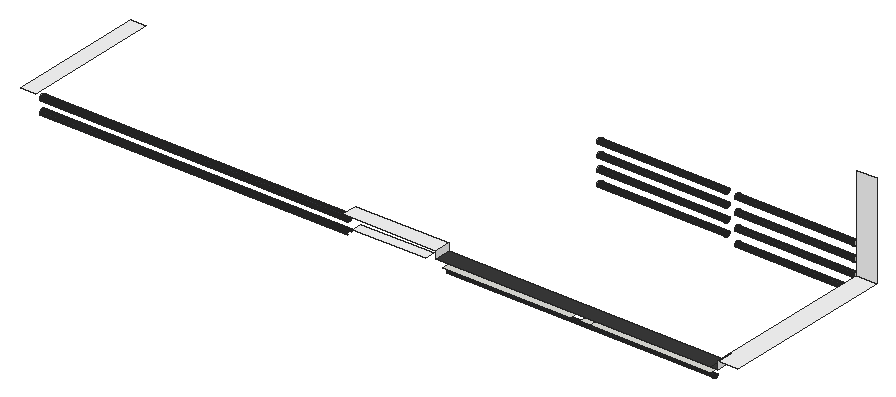
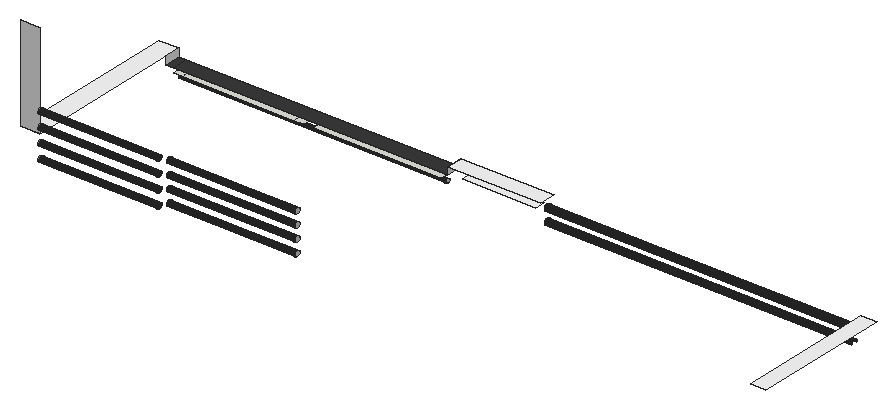
# SketchUp Ruby script. Lengths in inches.
U = 1.inch
M = Sketchup.active_model
def pt(a) = Geom::Point3d.new(a.map { |v| v * U })
def face(e, loops, mat)
  f = e.add_face(loops[0].map { |a| pt(a) })
  loops[1..].each { |l| e.add_face(l.map { |a| pt(a) }).erase! }
  f.material = f.back_material = mat if mat
  f
end
# faces: each face lists its corners as indices into pts; further lists are holes
def faces(e, pts, list, mat = nil) = list.each { |f| face(e, (f[0].is_a?(Array) ? f : [f]).map { |l| l.map { |i| pts[i] } }, mat) }
# xy, xz, yz: faces in a plane at the given z, y or x. An outline is a flat list of corners, or four numbers for a rectangle; further outlines are holes
def ring(l) = l.size == 4 ? [[l[0], l[1]], [l[2], l[1]], [l[2], l[3]], [l[0], l[3]]] : l.each_slice(2).to_a
def flat(e, list, mat, &to3) = list.each { |f| face(e, (f[0].is_a?(Array) ? f : [f]).map { |l| ring(l).map { |u, v| to3.(u, v) } }, mat) }
def xy(e, z, list, mat = nil) = flat(e, list, mat) { |x, y| [x, y, z] }
def xz(e, y, list, mat = nil) = flat(e, list, mat) { |x, z| [x, y, z] }
def yz(e, x, list, mat = nil) = flat(e, list, mat) { |y, z| [x, y, z] }
def lines(e, pts, list) = list.each { |a, b| e.add_line(pt(pts[a]), pt(pts[b])) }
# prism: a flat outline (further loops are holes) pulled along v
def prism(e, loops, v, mat = nil)
  f = face(e, loops, mat); d = Geom::Vector3d.new(v.map { |x| x * U })
  f.pushpull(f.normal.samedirection?(d) ? d.length : -d.length)
end
def box(e, o, s, mat = nil) = prism(e, [[o, [o[0] + s[0], o[1], o[2]], [o[0] + s[0], o[1] + s[1], o[2]], [o[0], o[1] + s[1], o[2]]]], [0, 0, s[2]], mat)
def at(x, y, z, deg = 0) = Geom::Transformation.translation(pt([x, y, z])) * Geom::Transformation.rotation(ORIGIN, Z_AXIS, deg.degrees)
def axes(o, x, y, z) = Geom::Transformation.new([*x, 0, *y, 0, *z, 0, *pt(o).to_a, 1])
def part(name) = M.definitions.add(name)
# library, detail: a bought-in or finely detailed component or shape, given as its bounding box
def library(name, o, s) = part(name).tap { |d| box(d.entities, o, s) }
def detail(e, o, s) = box(e.add_group.entities, o, s)
def put(e, d, t, mat = nil) = e.add_instance(d, t).tap { |i| i.material = mat if mat }
def group(e, t, mat = nil) = e.add_group.tap { |g| g.transformation = t; g.material = mat if mat }.entities
root = M.entities
M.materials.add("[Carrera Marble]").color = [252, 252, 252]
M.materials.add("[Color M07]").color = [58, 58, 58]
M.materials.add("[Formica Laminate Dark]").color = [50, 53, 60]
xy(root,65.34,[[464.36,270.82,564.04,283.23],[571.61,270.82,579.17,283.23],[579.17,270.82,673.42,283.23]])
xy(root,67.32,[[394.4,270.82,451.35,278.69]],"[Carrera Marble]")
xy(root,69.375,[[459.28,270.82,673.42,283.23],[673.42,270.82,679.23,283.23]],"[Color M07]")
xy(root,75.25,[[134.55,270.82,146.33,378.85],[386.47,270.82,459.28,283.23],[679.23,270.82,694.52,406.29]],"[Carrera Marble]")
xz(root,406.29,[[679.23,75.25,694.52,149.125]],"[Carrera Marble]")
yz(root,146.33,[[277.43,67.33,276.8,67.41,276.21,67.65,275.71,68.04,275.32,68.54,275.08,69.13,274.99,69.76,275.08,70.39,275.32,70.98,275.71,71.49,276.21,71.875,276.8,72.12,277.43,72.2,278.0625,72.12,278.65,71.875,279.15,71.49,279.54,70.98,279.78,70.39,279.87,69.76,279.78,69.13,279.54,68.54,279.15,68.04,278.65,67.65,278.0625,67.41]])
yz(root,459.28,[[270.82,69.375,283.23,75.25]],"[Carrera Marble]")
yz(root,464.36,[[276.43,59.2,276.06,59.25,275.71,59.4,275.41,59.625,275.18,59.92,275.04,60.27,274.99,60.64,275.04,61.01,275.18,61.36,275.41,61.66,275.71,61.89,276.06,62.03,276.43,62.08,276.8,62.03,277.15,61.89,277.44,61.66,277.67,61.36,277.82,61.01,277.87,60.64,277.82,60.27,277.67,59.92,277.44,59.625,277.15,59.4,276.8,59.25]])
yz(root,473.77,[[411.5,63.75,411,63.8125,410.53,64.01,410.13,64.32,409.82,64.72,409.63,65.18,409.5625,65.6875,409.63,66.1875,409.82,66.65,410.13,67.06,410.53,67.36,411,67.56,411.5,67.625,412,67.56,412.47,67.36,412.87,67.06,413.18,66.65,413.37,66.1875,413.4375,65.6875,413.37,65.18,413.18,64.72,412.87,64.32,412.47,64.01,412,63.8125],[411.5,73.75,411,73.8125,410.53,74.01,410.13,74.32,409.82,74.72,409.63,75.18,409.5625,75.6875,409.63,76.1875,409.82,76.65,410.13,77.06,410.53,77.36,411,77.56,411.5,77.625,412,77.56,412.47,77.36,412.87,77.06,413.18,76.65,413.37,76.1875,413.4375,75.6875,413.37,75.18,413.18,74.72,412.87,74.32,412.47,74.01,412,73.8125],[411.5,83.75,411,83.8125,410.53,84.01,410.13,84.32,409.82,84.72,409.63,85.18,409.5625,85.6875,409.63,86.1875,409.82,86.65,410.13,87.06,410.53,87.36,411,87.56,411.5,87.625,412,87.56,412.47,87.36,412.87,87.06,413.18,86.65,413.37,86.1875,413.4375,85.6875,413.37,85.18,413.18,84.72,412.87,84.32,412.47,84.01,412,83.8125],[411.5,93.75,411,93.8125,410.53,94.01,410.13,94.32,409.82,94.72,409.63,95.18,409.5625,95.6875,409.63,96.1875,409.82,96.65,410.13,97.06,410.53,97.36,411,97.56,411.5,97.625,412,97.56,412.47,97.36,412.87,97.06,413.18,96.65,413.37,96.1875,413.4375,95.6875,413.37,95.18,413.18,94.72,412.87,94.32,412.47,94.01,412,93.8125]])
yz(root,674.94,[[411.43,59.33,411.93,59.4,412.39,59.59,412.8,59.9,413.1,60.3,413.3,60.77,413.36,61.27,413.3,61.77,413.1,62.24,412.8,62.64,412.39,62.95,411.93,63.14,411.43,63.21,410.92,63.14,410.46,62.95,410.06,62.64,409.75,62.24,409.55,61.77,409.49,61.27,409.55,60.77,409.75,60.3,410.06,59.9,410.46,59.59,410.92,59.4],[411.43,70.46,411.93,70.52,412.39,70.72,412.8,71.02,413.1,71.43,413.3,71.89,413.36,72.39,413.3,72.9,413.1,73.36,412.8,73.76,412.39,74.07,411.93,74.27,411.43,74.33,410.92,74.27,410.46,74.07,410.06,73.76,409.75,73.36,409.55,72.9,409.49,72.39,409.55,71.89,409.75,71.43,410.06,71.02,410.46,70.72,410.92,70.52],[411.43,81.58,411.93,81.65,412.39,81.84,412.8,82.15,413.1,82.55,413.3,83.02,413.36,83.52,413.3,84.02,413.1,84.49,412.8,84.89,412.39,85.2,411.93,85.39,411.43,85.46,410.92,85.39,410.46,85.2,410.06,84.89,409.75,84.49,409.55,84.02,409.49,83.52,409.55,83.02,409.75,82.55,410.06,82.15,410.46,81.84,410.92,81.65],[411.43,92.71,411.93,92.77,412.39,92.97,412.8,93.27,413.1,93.68,413.3,94.14,413.36,94.64,413.3,95.15,413.1,95.61,412.8,96.01,412.39,96.32,411.93,96.52,411.43,96.58,410.92,96.52,410.46,96.32,410.06,96.01,409.75,95.61,409.55,95.15,409.49,94.64,409.55,94.14,409.75,93.68,410.06,93.27,410.46,92.97,410.92,92.77]])
yz(root,679.23,[[270.82,69.375,283.23,75.25]],"[Carrera Marble]")
p = [[146.33,274.99,59.45],[146.33,275.08,58.82],[386.47,275.08,58.82],[386.47,274.99,59.45],[146.33,279.78,58.82],[146.33,279.87,59.45],
  [386.47,279.87,59.45],[386.47,279.78,58.82],[464.36,276.06,59.25],[464.36,276.43,59.2],[673.42,276.43,59.2],[673.42,276.06,59.25],
  [464.36,276.8,59.25],[673.42,276.8,59.25],[464.36,275.71,59.4],[673.42,275.71,59.4],[464.36,277.15,59.4],[673.42,277.15,59.4],
  [674.94,411.43,59.33],[674.94,410.92,59.4],[581.54,410.92,59.4],[581.54,411.43,59.33],[674.94,411.93,59.4],[581.54,411.93,59.4],
  [464.36,275.41,59.625],[673.42,275.41,59.625],[464.36,277.44,59.625],[673.42,277.44,59.625],[674.94,410.46,59.59],[581.54,410.46,59.59],
  [674.94,412.39,59.59],[581.54,412.39,59.59],[146.33,275.08,60.08],[386.47,275.08,60.08],[146.33,279.78,60.08],[386.47,279.78,60.08],
  [464.36,275.18,59.92],[673.42,275.18,59.92],[464.36,277.67,59.92],[673.42,277.67,59.92],[674.94,410.06,59.9],[581.54,410.06,59.9],
  [674.94,412.8,59.9],[581.54,412.8,59.9],[464.36,275.04,60.27],[673.42,275.04,60.27],[464.36,277.82,60.27],[673.42,277.82,60.27],
  [674.94,409.75,60.3],[581.54,409.75,60.3],[674.94,413.1,60.3],[581.54,413.1,60.3],[146.33,275.32,60.67],[386.47,275.32,60.67],
  [146.33,279.54,60.67],[386.47,279.54,60.67],[464.36,274.99,60.64],[673.42,274.99,60.64],[464.36,277.87,60.64],[673.42,277.87,60.64],
  [674.94,409.55,60.77],[581.54,409.55,60.77],[674.94,413.3,60.77],[581.54,413.3,60.77],[464.36,275.04,61.01],[673.42,275.04,61.01],
  [464.36,277.82,61.01],[673.42,277.82,61.01],[146.33,275.71,61.17],[386.47,275.71,61.17],[146.33,279.15,61.17],[386.47,279.15,61.17],
  [674.94,409.49,61.27],[581.54,409.49,61.27],[674.94,413.36,61.27],[581.54,413.36,61.27],[464.36,275.18,61.36],[673.42,275.18,61.36],
  [464.36,277.67,61.36],[673.42,277.67,61.36],[146.33,276.21,61.5625],[386.47,276.21,61.5625],[146.33,278.65,61.5625],[386.47,278.65,61.5625],
  [674.94,409.55,61.77],[581.54,409.55,61.77],[674.94,413.3,61.77],[581.54,413.3,61.77],[464.36,275.41,61.66],[673.42,275.41,61.66],
  [464.36,277.44,61.66],[673.42,277.44,61.66],[146.33,276.8,61.8],[386.47,276.8,61.8],[146.33,278.0625,61.8],[386.47,278.0625,61.8],
  [464.36,275.71,61.89],[673.42,275.71,61.89],[464.36,277.15,61.89],[673.42,277.15,61.89],[146.33,277.43,61.89],[386.47,277.43,61.89],
  [674.94,409.75,62.24],[581.54,409.75,62.24],[674.94,413.1,62.24],[581.54,413.1,62.24],[464.36,276.06,62.03],[673.42,276.06,62.03],
  [464.36,276.8,62.03],[673.42,276.8,62.03],[464.36,276.43,62.08],[673.42,276.43,62.08],[674.94,410.06,62.64],[581.54,410.06,62.64],
  [674.94,412.8,62.64],[581.54,412.8,62.64],[674.94,410.46,62.95],[581.54,410.46,62.95],[674.94,412.39,62.95],[581.54,412.39,62.95],
  [674.94,410.92,63.14],[581.54,410.92,63.14],[674.94,411.93,63.14],[581.54,411.93,63.14],[674.94,411.43,63.21],[581.54,411.43,63.21],
  [473.77,411,63.8125],[473.77,411.5,63.75],[574.36,411.5,63.75],[574.36,411,63.8125],[473.77,412,63.8125],[574.36,412,63.8125],
  [473.77,410.53,64.01],[574.36,410.53,64.01],[473.77,412.47,64.01],[574.36,412.47,64.01],[473.77,410.13,64.32],[574.36,410.13,64.32],
  [473.77,412.87,64.32],[574.36,412.87,64.32],[473.77,409.82,64.72],[574.36,409.82,64.72],[473.77,413.18,64.72],[574.36,413.18,64.72],
  [473.77,409.63,65.18],[574.36,409.63,65.18],[473.77,413.37,65.18],[574.36,413.37,65.18],[473.77,409.5625,65.6875],[574.36,409.5625,65.6875],
  [473.77,413.4375,65.6875],[574.36,413.4375,65.6875],[473.77,409.63,66.1875],[574.36,409.63,66.1875],[473.77,413.37,66.1875],[574.36,413.37,66.1875],
  [473.77,409.82,66.65],[574.36,409.82,66.65],[473.77,413.18,66.65],[574.36,413.18,66.65],[473.77,410.13,67.06],[574.36,410.13,67.06],
  [473.77,412.87,67.06],[574.36,412.87,67.06],[473.77,410.53,67.36],[574.36,410.53,67.36],[473.77,412.47,67.36],[574.36,412.47,67.36],
  [146.33,276.8,67.41],[146.33,277.43,67.33],[386.47,277.43,67.33],[386.47,276.8,67.41],[146.33,278.0625,67.41],[386.47,278.0625,67.41],
  [146.33,276.21,67.65],[386.47,276.21,67.65],[146.33,278.65,67.65],[386.47,278.65,67.65],[473.77,411,67.56],[574.36,411,67.56],
  [473.77,412,67.56],[574.36,412,67.56],[473.77,411.5,67.625],[574.36,411.5,67.625],[146.33,275.71,68.04],[386.47,275.71,68.04],
  [146.33,279.15,68.04],[386.47,279.15,68.04],[146.33,275.32,68.54],[386.47,275.32,68.54],[146.33,279.54,68.54],[386.47,279.54,68.54],
  [146.33,275.08,69.13],[386.47,275.08,69.13],[146.33,279.78,69.13],[386.47,279.78,69.13],[146.33,274.99,69.76],[386.47,274.99,69.76],
  [146.33,279.87,69.76],[386.47,279.87,69.76],[146.33,275.08,70.39],[386.47,275.08,70.39],[146.33,279.78,70.39],[386.47,279.78,70.39],
  [146.33,275.32,70.98],[386.47,275.32,70.98],[146.33,279.54,70.98],[386.47,279.54,70.98],[674.94,410.92,70.52],[674.94,410.46,70.72],
  [581.54,410.46,70.72],[581.54,410.92,70.52],[674.94,411.43,70.46],[581.54,411.43,70.46],[674.94,411.93,70.52],[581.54,411.93,70.52],
  [674.94,412.39,70.72],[581.54,412.39,70.72],[674.94,410.06,71.02],[581.54,410.06,71.02],[674.94,412.8,71.02],[581.54,412.8,71.02],
  [146.33,275.71,71.49],[386.47,275.71,71.49],[146.33,279.15,71.49],[386.47,279.15,71.49],[674.94,409.75,71.43],[581.54,409.75,71.43],
  [674.94,413.1,71.43],[581.54,413.1,71.43],[674.94,409.55,71.89],[581.54,409.55,71.89],[674.94,413.3,71.89],[581.54,413.3,71.89],
  [146.33,276.21,71.875],[386.47,276.21,71.875],[146.33,278.65,71.875],[386.47,278.65,71.875],[146.33,276.8,72.12],[386.47,276.8,72.12],
  [146.33,278.0625,72.12],[386.47,278.0625,72.12],[674.94,409.49,72.39],[581.54,409.49,72.39],[674.94,413.36,72.39],[581.54,413.36,72.39],
  [146.33,277.43,72.2],[386.47,277.43,72.2],[674.94,409.55,72.9],[581.54,409.55,72.9],[674.94,413.3,72.9],[581.54,413.3,72.9],
  [674.94,409.75,73.36],[581.54,409.75,73.36],[674.94,413.1,73.36],[581.54,413.1,73.36],[674.94,410.06,73.76],[581.54,410.06,73.76],
  [674.94,412.8,73.76],[581.54,412.8,73.76],[473.77,411,73.8125],[473.77,411.5,73.75],[574.36,411.5,73.75],[574.36,411,73.8125],
  [473.77,412,73.8125],[574.36,412,73.8125],[674.94,410.46,74.07],[581.54,410.46,74.07],[473.77,410.53,74.01],[574.36,410.53,74.01],
  [473.77,412.47,74.01],[574.36,412.47,74.01],[674.94,412.39,74.07],[581.54,412.39,74.07],[473.77,410.13,74.32],[574.36,410.13,74.32],
  [473.77,412.87,74.32],[574.36,412.87,74.32],[674.94,410.92,74.27],[581.54,410.92,74.27],[674.94,411.93,74.27],[581.54,411.93,74.27],
  [473.77,409.82,74.72],[574.36,409.82,74.72],[674.94,411.43,74.33],[581.54,411.43,74.33],[473.77,413.18,74.72],[574.36,413.18,74.72],
  [473.77,409.63,75.18],[574.36,409.63,75.18],[473.77,413.37,75.18],[574.36,413.37,75.18],[473.77,409.5625,75.6875],[574.36,409.5625,75.6875],
  [473.77,413.4375,75.6875],[574.36,413.4375,75.6875],[473.77,409.63,76.1875],[574.36,409.63,76.1875],[473.77,413.37,76.1875],[574.36,413.37,76.1875],
  [473.77,409.82,76.65],[574.36,409.82,76.65],[473.77,413.18,76.65],[574.36,413.18,76.65],[473.77,410.13,77.06],[574.36,410.13,77.06],
  [473.77,412.87,77.06],[574.36,412.87,77.06],[473.77,410.53,77.36],[574.36,410.53,77.36],[473.77,412.47,77.36],[574.36,412.47,77.36],
  [473.77,411,77.56],[574.36,411,77.56],[473.77,412,77.56],[574.36,412,77.56],[473.77,411.5,77.625],[574.36,411.5,77.625],
  [674.94,410.92,81.65],[674.94,410.46,81.84],[581.54,410.46,81.84],[581.54,410.92,81.65],[674.94,411.43,81.58],[581.54,411.43,81.58],
  [674.94,411.93,81.65],[581.54,411.93,81.65],[674.94,412.39,81.84],[581.54,412.39,81.84],[674.94,410.06,82.15],[581.54,410.06,82.15],
  [674.94,412.8,82.15],[581.54,412.8,82.15],[674.94,409.75,82.55],[581.54,409.75,82.55],[674.94,413.1,82.55],[581.54,413.1,82.55],
  [674.94,409.55,83.02],[581.54,409.55,83.02],[674.94,413.3,83.02],[581.54,413.3,83.02],[674.94,409.49,83.52],[581.54,409.49,83.52],
  [674.94,413.36,83.52],[581.54,413.36,83.52],[674.94,409.55,84.02],[581.54,409.55,84.02],[674.94,413.3,84.02],[581.54,413.3,84.02],
  [473.77,411,83.8125],[473.77,411.5,83.75],[574.36,411.5,83.75],[574.36,411,83.8125],[473.77,412,83.8125],[574.36,412,83.8125],
  [473.77,410.53,84.01],[574.36,410.53,84.01],[473.77,412.47,84.01],[574.36,412.47,84.01],[674.94,409.75,84.49],[581.54,409.75,84.49],
  [473.77,410.13,84.32],[574.36,410.13,84.32],[473.77,412.87,84.32],[574.36,412.87,84.32],[674.94,413.1,84.49],[581.54,413.1,84.49],
  [473.77,409.82,84.72],[574.36,409.82,84.72],[473.77,413.18,84.72],[574.36,413.18,84.72],[674.94,410.06,84.89],[581.54,410.06,84.89],
  [674.94,412.8,84.89],[581.54,412.8,84.89],[473.77,409.63,85.18],[574.36,409.63,85.18],[473.77,413.37,85.18],[574.36,413.37,85.18],
  [674.94,410.46,85.2],[581.54,410.46,85.2],[674.94,412.39,85.2],[581.54,412.39,85.2],[473.77,409.5625,85.6875],[574.36,409.5625,85.6875],
  [674.94,410.92,85.39],[581.54,410.92,85.39],[674.94,411.93,85.39],[581.54,411.93,85.39],[473.77,413.4375,85.6875],[574.36,413.4375,85.6875],
  [674.94,411.43,85.46],[581.54,411.43,85.46],[473.77,409.63,86.1875],[574.36,409.63,86.1875],[473.77,413.37,86.1875],[574.36,413.37,86.1875],
  [473.77,409.82,86.65],[574.36,409.82,86.65],[473.77,413.18,86.65],[574.36,413.18,86.65],[473.77,410.13,87.06],[574.36,410.13,87.06],
  [473.77,412.87,87.06],[574.36,412.87,87.06],[473.77,410.53,87.36],[574.36,410.53,87.36],[473.77,412.47,87.36],[574.36,412.47,87.36],
  [473.77,411,87.56],[574.36,411,87.56],[473.77,412,87.56],[574.36,412,87.56],[473.77,411.5,87.625],[574.36,411.5,87.625],
  [674.94,411.43,92.71],[674.94,410.92,92.77],[581.54,410.92,92.77],[581.54,411.43,92.71],[674.94,411.93,92.77],[581.54,411.93,92.77],
  [674.94,410.46,92.97],[581.54,410.46,92.97],[674.94,412.39,92.97],[581.54,412.39,92.97],[674.94,410.06,93.27],[581.54,410.06,93.27],
  [674.94,412.8,93.27],[581.54,412.8,93.27],[674.94,409.75,93.68],[581.54,409.75,93.68],[674.94,413.1,93.68],[581.54,413.1,93.68],
  [674.94,409.55,94.14],[581.54,409.55,94.14],[473.77,411,93.8125],[473.77,411.5,93.75],[574.36,411.5,93.75],[574.36,411,93.8125],
  [473.77,412,93.8125],[574.36,412,93.8125],[674.94,413.3,94.14],[581.54,413.3,94.14],[473.77,410.53,94.01],[574.36,410.53,94.01],
  [473.77,412.47,94.01],[574.36,412.47,94.01],[473.77,410.13,94.32],[574.36,410.13,94.32],[473.77,412.87,94.32],[574.36,412.87,94.32],
  [674.94,409.49,94.64],[581.54,409.49,94.64],[674.94,413.36,94.64],[581.54,413.36,94.64],[473.77,409.82,94.72],[574.36,409.82,94.72],
  [473.77,413.18,94.72],[574.36,413.18,94.72],[674.94,409.55,95.15],[581.54,409.55,95.15],[674.94,413.3,95.15],[581.54,413.3,95.15],
  [473.77,409.63,95.18],[574.36,409.63,95.18],[473.77,413.37,95.18],[574.36,413.37,95.18],[674.94,409.75,95.61],[581.54,409.75,95.61],
  [674.94,413.1,95.61],[581.54,413.1,95.61],[473.77,409.5625,95.6875],[574.36,409.5625,95.6875],[473.77,413.4375,95.6875],[574.36,413.4375,95.6875],
  [674.94,410.06,96.01],[581.54,410.06,96.01],[674.94,412.8,96.01],[581.54,412.8,96.01],[473.77,409.63,96.1875],[574.36,409.63,96.1875],
  [473.77,413.37,96.1875],[574.36,413.37,96.1875],[674.94,410.46,96.32],[581.54,410.46,96.32],[674.94,412.39,96.32],[581.54,412.39,96.32],
  [473.77,409.82,96.65],[574.36,409.82,96.65],[473.77,413.18,96.65],[574.36,413.18,96.65],[674.94,410.92,96.52],[581.54,410.92,96.52],
  [674.94,411.93,96.52],[581.54,411.93,96.52],[674.94,411.43,96.58],[581.54,411.43,96.58],[473.77,410.13,97.06],[574.36,410.13,97.06],
  [473.77,412.87,97.06],[574.36,412.87,97.06],[473.77,410.53,97.36],[574.36,410.53,97.36],[473.77,412.47,97.36],[574.36,412.47,97.36],
  [473.77,411,97.56],[574.36,411,97.56],[473.77,412,97.56],[574.36,412,97.56],[473.77,411.5,97.625],[574.36,411.5,97.625]]
faces(root,p,[[0,1,2,3],[4,5,6,7],[8,9,10,11],[9,12,13,10],[14,8,11,15],[12,16,17,13],[24,14,15,25],[16,26,27,17],
  [32,0,3,33],[5,34,35,6],[36,24,25,37],[26,38,39,27],[44,36,37,45],[38,46,47,39],[52,32,33,53],[34,54,55,35],
  [56,44,45,57],[46,58,59,47],[64,56,57,65],[58,66,67,59],[68,52,53,69],[54,70,71,55],[76,64,65,77],[66,78,79,67],
  [80,68,69,81],[70,82,83,71],[88,76,77,89],[78,90,91,79],[92,80,81,93],[82,94,95,83],[96,88,89,97],[90,98,99,91],
  [100,92,93,101],[94,100,101,95],[106,96,97,107],[98,108,109,99],[110,106,107,111],[108,110,111,109],[168,169,170,171],[169,172,173,170],
  [174,168,171,175],[172,176,177,173],[184,174,175,185],[176,186,187,177],[188,184,185,189],[186,190,191,187],[192,188,189,193],[190,194,195,191],
  [196,192,193,197],[194,198,199,195],[200,196,197,201],[198,202,203,199],[204,200,201,205],[202,206,207,203],[222,204,205,223],[206,224,225,207],
  [234,222,223,235],[224,236,237,225],[238,234,235,239],[236,240,241,237],[246,238,239,247],[240,246,247,241]],"[Formica Laminate Dark]")
faces(root,p,[[18,19,20,21],[22,18,21,23],[19,28,29,20],[30,22,23,31],[28,40,41,29],[42,30,31,43],[40,48,49,41],[50,42,43,51],
  [48,60,61,49],[62,50,51,63],[60,72,73,61],[74,62,63,75],[72,84,85,73],[86,74,75,87],[84,102,103,85],[104,86,87,105],
  [102,112,113,103],[114,104,105,115],[112,116,117,113],[118,114,115,119],[116,120,121,117],[122,118,119,123],[120,124,125,121],[124,122,123,125],
  [126,127,128,129],[127,130,131,128],[132,126,129,133],[130,134,135,131],[136,132,133,137],[134,138,139,135],[140,136,137,141],[138,142,143,139],
  [144,140,141,145],[142,146,147,143],[148,144,145,149],[146,150,151,147],[152,148,149,153],[150,154,155,151],[156,152,153,157],[154,158,159,155],
  [160,156,157,161],[158,162,163,159],[164,160,161,165],[162,166,167,163],[178,164,165,179],[166,180,181,167],[182,178,179,183],[180,182,183,181],
  [208,209,210,211],[212,208,211,213],[214,212,213,215],[216,214,215,217],[209,218,219,210],[220,216,217,221],[218,226,227,219],[228,220,221,229],
  [226,230,231,227],[232,228,229,233],[230,242,243,231],[244,232,233,245],[242,248,249,243],[250,244,245,251],[248,252,253,249],[254,250,251,255],
  [252,256,257,253],[258,254,255,259],[260,261,262,263],[261,264,265,262],[256,266,267,257],[268,260,263,269],[264,270,271,265],[272,258,259,273],
  [274,268,269,275],[270,276,277,271],[266,278,279,267],[280,272,273,281],[282,274,275,283],[278,284,285,279],[284,280,281,285],[276,286,287,277],
  [288,282,283,289],[286,290,291,287],[292,288,289,293],[290,294,295,291],[296,292,293,297],[294,298,299,295],[300,296,297,301],[298,302,303,299],
  [304,300,301,305],[302,306,307,303],[308,304,305,309],[306,310,311,307],[312,308,309,313],[310,314,315,311],[316,312,313,317],[314,316,317,315],
  [318,319,320,321],[322,318,321,323],[324,322,323,325],[326,324,325,327],[319,328,329,320],[330,326,327,331],[328,332,333,329],[334,330,331,335],
  [332,336,337,333],[338,334,335,339],[336,340,341,337],[342,338,339,343],[340,344,345,341],[346,342,343,347],[348,349,350,351],[349,352,353,350],
  [354,348,351,355],[352,356,357,353],[344,358,359,345],[360,354,355,361],[356,362,363,357],[364,346,347,365],[366,360,361,367],[362,368,369,363],
  [358,370,371,359],[372,364,365,373],[374,366,367,375],[368,376,377,369],[370,378,379,371],[380,372,373,381],[382,374,375,383],[378,384,385,379],
  [386,380,381,387],[376,388,389,377],[384,390,391,385],[390,386,387,391],[392,382,383,393],[388,394,395,389],[396,392,393,397],[394,398,399,395],
  [400,396,397,401],[398,402,403,399],[404,400,401,405],[402,406,407,403],[408,404,405,409],[406,410,411,407],[412,408,409,413],[410,412,413,411],
  [414,415,416,417],[418,414,417,419],[415,420,421,416],[422,418,419,423],[420,424,425,421],[426,422,423,427],[424,428,429,425],[430,426,427,431],
  [428,432,433,429],[434,435,436,437],[435,438,439,436],[440,430,431,441],[442,434,437,443],[438,444,445,439],[446,442,443,447],[444,448,449,445],
  [432,450,451,433],[452,440,441,453],[454,446,447,455],[448,456,457,449],[450,458,459,451],[460,452,453,461],[462,454,455,463],[456,464,465,457],
  [458,466,467,459],[468,460,461,469],[470,462,463,471],[464,472,473,465],[466,474,475,467],[476,468,469,477],[478,470,471,479],[472,480,481,473],
  [474,482,483,475],[484,476,477,485],[486,478,479,487],[480,488,489,481],[482,490,491,483],[492,484,485,493],[490,494,495,491],[494,492,493,495],
  [496,486,487,497],[488,498,499,489],[500,496,497,501],[498,502,503,499],[504,500,501,505],[502,506,507,503],[508,504,505,509],[506,508,509,507]],"[Color M07]")
